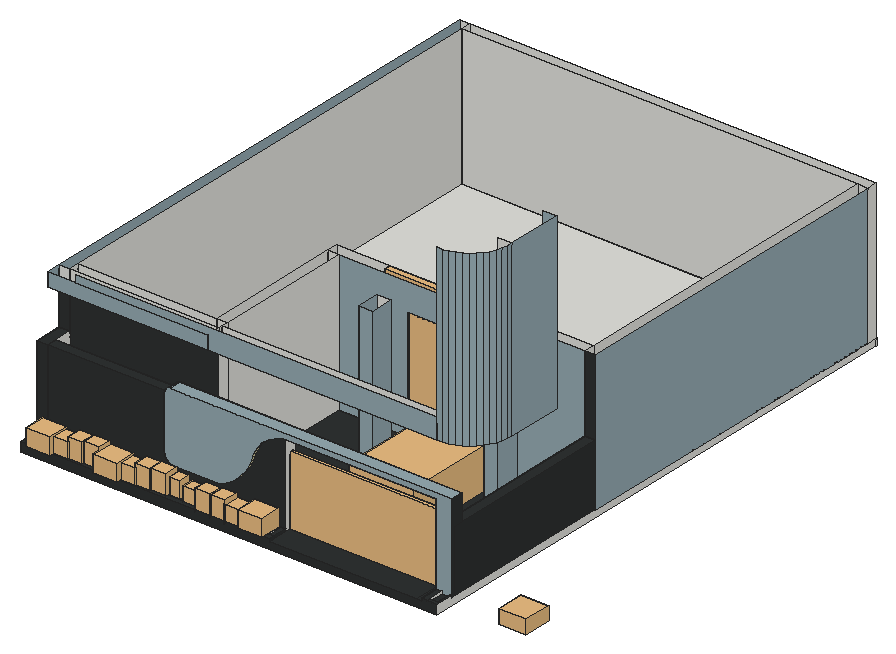
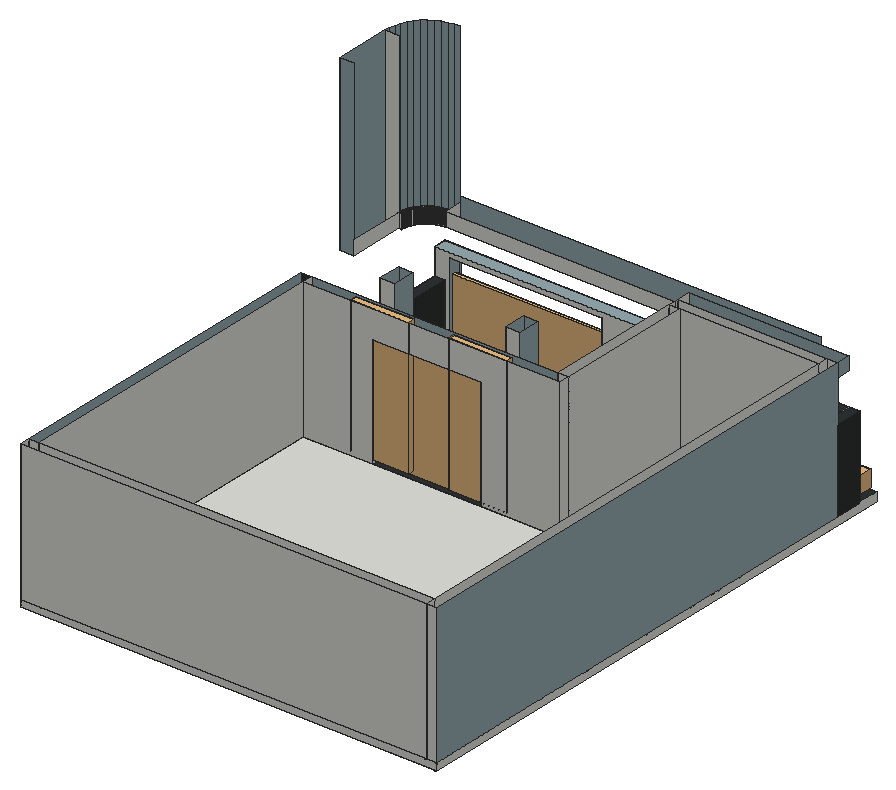
# SketchUp Ruby script. Lengths in inches.
U = 1.inch
M = Sketchup.active_model
def pt(a) = Geom::Point3d.new(a.map { |v| v * U })
def face(e, loops, mat)
  f = e.add_face(loops[0].map { |a| pt(a) })
  loops[1..].each { |l| e.add_face(l.map { |a| pt(a) }).erase! }
  f.material = f.back_material = mat if mat
  f
end
# faces: each face lists its corners as indices into pts; further lists are holes
def faces(e, pts, list, mat = nil) = list.each { |f| face(e, (f[0].is_a?(Array) ? f : [f]).map { |l| l.map { |i| pts[i] } }, mat) }
# xy, xz, yz: faces in a plane at the given z, y or x. An outline is a flat list of corners, or four numbers for a rectangle; further outlines are holes
def ring(l) = l.size == 4 ? [[l[0], l[1]], [l[2], l[1]], [l[2], l[3]], [l[0], l[3]]] : l.each_slice(2).to_a
def flat(e, list, mat, &to3) = list.each { |f| face(e, (f[0].is_a?(Array) ? f : [f]).map { |l| ring(l).map { |u, v| to3.(u, v) } }, mat) }
def xy(e, z, list, mat = nil) = flat(e, list, mat) { |x, y| [x, y, z] }
def xz(e, y, list, mat = nil) = flat(e, list, mat) { |x, z| [x, y, z] }
def yz(e, x, list, mat = nil) = flat(e, list, mat) { |y, z| [x, y, z] }
def lines(e, pts, list) = list.each { |a, b| e.add_line(pt(pts[a]), pt(pts[b])) }
# prism: a flat outline (further loops are holes) pulled along v
def prism(e, loops, v, mat = nil)
  f = face(e, loops, mat); d = Geom::Vector3d.new(v.map { |x| x * U })
  f.pushpull(f.normal.samedirection?(d) ? d.length : -d.length)
end
def box(e, o, s, mat = nil) = prism(e, [[o, [o[0] + s[0], o[1], o[2]], [o[0] + s[0], o[1] + s[1], o[2]], [o[0], o[1] + s[1], o[2]]]], [0, 0, s[2]], mat)
def at(x, y, z, deg = 0) = Geom::Transformation.translation(pt([x, y, z])) * Geom::Transformation.rotation(ORIGIN, Z_AXIS, deg.degrees)
def axes(o, x, y, z) = Geom::Transformation.new([*x, 0, *y, 0, *z, 0, *pt(o).to_a, 1])
def part(name) = M.definitions.add(name)
# library, detail: a bought-in or finely detailed component or shape, given as its bounding box
def library(name, o, s) = part(name).tap { |d| box(d.entities, o, s) }
def detail(e, o, s) = box(e.add_group.entities, o, s)
def put(e, d, t, mat = nil) = e.add_instance(d, t).tap { |i| i.material = mat if mat }
def group(e, t, mat = nil) = e.add_group.tap { |g| g.transformation = t; g.material = mat if mat }.entities
root = M.entities
M.materials.add("Emissive").color = [234, 228, 175]
M.materials.add("Generic").color = [150, 171, 178]
M.materials.add("Generic\#1").color = [47, 50, 50]
c1 = library("Potted Plant 50-12",[-6.11,-5.26,0],[11.24,10.56,13.41])
c2 = library("Untitled",[332.1875,126.3,0],[192,3,60])
c3 = library("2016+Honda+Civic+LX+Sedan",[0.01,0.03,0.02],[16.17,34.46,10.62])
c4 = library("Window 46-47",[-61.02,-2.17,0],[122.04,4.34,74.02])
c5 = library("Potted Plant 50-23",[-3.4,-3.5,0],[6.8,7,9.93])
c6 = library("Plant 160 012",[-4.91,-4.04,0],[10.03,8.97,14.29])
c7 = library("Erigeron glaucus 001",[-10.99,-11.02,0],[21.02,20.18,22.01])
c8 = library("Erigeron glaucus 004",[-15.59,-14.45,0.01],[31.39,28.46,21.32])
c9 = library("Ficus elastica Belize 002",[-7.92,-8.8125,0.01],[22.14,24.73,36.43])
c10 = library("Curtains 003",[-24.98,-2.79,0.01],[49.96,5.58,117.31])
c11 = library("Dome Light",[-12,-12,0],[24,24,12])
xy(root,-6,[[1.218,0,361.218,474.0625],[1.218,474.0625,361.218,474.3125]])
xy(root,0,[[1.218,18.0625,10.218,42.0625],[10.218,18.0625,216.371,27.0625],[352.218,18.0625,361.218,171.0625],[10.218,27.0625,139.218,42.0625],[1.218,42.0625,10.218,474.0625],
  [10.218,42.0625,139.218,51.0625],[10.218,51.0625,130.218,51.0625,130.218,180.0625,352.218,180.0625,352.218,465.0625,10.218,465.0625],[130.218,51.0625,139.218,171.0625],[130.218,51.0625,139.218,51.0625,139.218,171.0625,199.218,171.0625,199.218,180.0625,130.218,180.0625],[130.218,171.0625,199.218,180.0625],
  [292.218,171.0625,352.218,180.0625],[352.218,171.0625,361.218,465.0625],[10.218,465.0625,361.218,474.0625],[1.218,474.0625,10.218,474.3125],[10.218,474.0625,361.218,474.3125]])
xy(root,0,[[[216.371,0,343.218,0,343.218,27.0625,352.218,27.0625,352.218,171.0625,292.218,171.0625,292.218,180.0625,199.218,180.0625,199.218,171.0625,139.218,171.0625,139.218,27.0625,216.371,27.0625],[194.174,124.131,206.361,143.851],[302.424,124.131,314.611,143.851]],[343.218,0,347.629,27.0625],[352.218,3.359,359.091,16],[10.218,5.216,211.73,18.0625]],"Generic\#1")
xy(root,1.8125,[[1.218,0,10.218,18.0625],[10.218,0,216.371,5.216],[211.73,5.216,216.371,18.0625]],"Generic\#1")
xy(root,2.1875,[[347.629,0,352.218,16],[352.218,0,361.218,3.359],[359.091,3.359,361.218,16]],"Generic\#1")
xy(root,18.134,[[121.177,16,159.058,18.0625]],"Emissive")
xy(root,54.125,[[352.218,18.0625,361.218,27.0625]])
xy(root,54.125,[[352.218,27.0625,361.218,171.0625]],"Generic\#1")
xy(root,72,[[1.218,18.0625,10.218,42.0625],[10.218,18.0625,112.749,27.0625]],"Generic\#1")
xy(root,72.458,[[216.371,16,347.629,18.0625],[216.371,18.0625,347.629,27.0625]],"Generic")
xy(root,76.875,[[118.243,16,361.218,27.0625]],"Generic")
xy(root,96,[[199.218,171.0625,292.218,180.0625]])
xy(root,108,[[139.218,29.933,1.206,30.0625,1.218,42.0625,139.218,41.933],[139.218,29.933,139.218,41.933,139.295,41.933,139.284,29.933],[337.222,41.748,337.218,42.0625,337.222,42.0625]])
xy(root,108,[[139.284,29.933,139.295,41.933,139.218,41.933,139.218,44.654,337.184,44.654,337.184,29.933],[337.218,29.933,337.218,42.0625,337.222,41.748,337.854,41.757,338.49,41.782,339.125,41.823,339.759,41.882,340.391,41.956,341.021,42.048,341.648,42.155,342.273,42.28,342.894,42.42,343.511,42.577,344.123,42.75,344.731,42.938,345.334,43.143,345.931,43.363,346.522,43.599,347.107,43.85,347.685,44.117,348.256,44.398,348.819,44.695,349.375,45.006,349.922,45.331,350.46,45.671,350.989,46.025,351.509,46.392,352.019,46.773,352.519,47.167,353.008,47.574,353.487,47.994,353.954,48.426,354.41,48.87,354.854,49.326,355.287,49.793,355.706,50.272,356.113,50.761,356.507,51.261,356.888,51.771,357.256,52.291,357.609,52.82,357.949,53.358,358.274,53.905,358.585,54.461,358.882,55.024,359.163,55.595,359.43,56.173,359.681,56.758,359.917,57.349,360.137,57.946,360.342,58.549,360.531,59.157,360.703,59.77,360.86,60.386,361,61.007,361.125,61.632,361.232,62.259,361.324,62.889,361.399,63.521,361.457,64.155,361.498,64.79,361.523,65.426,361.532,66.058,361.218,66.0625,373.218,66.0625,373.083,61.296,372.298,56.592,370.876,52.04,368.843,47.726,366.24,43.731,363.114,40.13,359.524,36.991,355.538,34.373,351.231,32.326,346.685,30.887,341.984,30.085],[337.222,41.748,337.222,42.0625,337.218,42.0625,337.184,44.654,337.778,44.662,338.338,44.684,338.897,44.72,339.455,44.772,340.012,44.838,340.567,44.918,341.119,45.013,341.669,45.122,342.215,45.246,342.758,45.384,343.298,45.536,343.833,45.702,344.364,45.882,344.89,46.076,345.41,46.284,345.925,46.505,346.434,46.74,346.937,46.988,347.433,47.249,347.922,47.523,348.403,47.809,348.877,48.108,349.343,48.42,349.801,48.743,350.25,49.078,350.69,49.425,351.121,49.784,351.542,50.153,351.954,50.534,352.355,50.925,352.746,51.326,353.127,51.738,353.496,52.159,353.855,52.59,354.202,53.03,354.537,53.479,354.861,53.937,355.172,54.403,355.471,54.877,355.757,55.358,356.031,55.847,356.292,56.343,356.54,56.846,356.775,57.355,356.996,57.87,357.204,58.391,357.398,58.916,357.578,59.447,357.744,59.982,357.896,60.522,358.034,61.065,358.158,61.612,358.267,62.161,358.362,62.714,358.442,63.268,358.508,63.825,358.56,64.383,358.596,64.942,358.618,65.502,358.626,66.096,361.218,66.0625,361.532,66.058,361.523,65.426,361.498,64.79,361.457,64.155,361.399,63.521,361.324,62.889,361.232,62.259,361.125,61.632,361,61.007,360.86,60.386,360.703,59.77,360.531,59.157,360.342,58.549,360.137,57.946,359.917,57.349,359.681,56.758,359.43,56.173,359.163,55.595,358.882,55.024,358.585,54.461,358.274,53.905,357.949,53.358,357.609,52.82,357.256,52.291,356.888,51.771,356.507,51.261,356.113,50.761,355.706,50.272,355.287,49.793,354.854,49.326,354.41,48.87,353.954,48.426,353.487,47.994,353.008,47.574,352.519,47.167,352.019,46.773,351.509,46.392,350.989,46.025,350.46,45.671,349.922,45.331,349.375,45.006,348.819,44.695,348.256,44.398,347.685,44.117,347.107,43.85,346.522,43.599,345.931,43.363,345.334,43.143,344.731,42.938,344.123,42.75,343.511,42.577,342.894,42.42,342.273,42.28,341.648,42.155,341.021,42.048,340.391,41.956,339.759,41.882,339.125,41.823,338.49,41.782,337.854,41.757],[361.218,66.0625,373.218,114.0625]],"Generic")
xz(root,0,[[1.218,-6,361.218,-6,361.218,2.1875,347.629,2.1875,347.629,0,216.371,0,216.371,1.8125,1.218,1.8125]],"Generic\#1")
xz(root,3.359,[[352.218,0,359.091,2.1875]])
xz(root,5.216,[[10.218,0,211.73,1.8125]])
xz(root,16,[[352.218,0,359.091,0,359.091,2.1875,361.218,2.1875,361.218,76.875,118.243,76.875,117.575,76.835,116.917,76.714,116.279,76.515,115.669,76.24,115.096,75.893,114.57,75.481,114.098,75.007,113.686,74.48,113.34,73.907,113.067,73.297,112.868,72.658,112.749,72,112.749,26.562,112.821,25.462,113.036,24.381,113.391,23.337,113.878,22.348,114.491,21.431,115.218,20.602,116.046,19.875,116.963,19.263,117.952,18.775,118.996,18.421,120.077,18.206,121.177,18.134,159.058,18.134,162.568,19.401,165.964,20.947,169.225,22.762,172.328,24.833,175.255,27.148,177.986,29.69,180.503,32.445,182.791,35.393,184.833,38.516,186.617,41.793,188.131,45.204,189.366,48.725,190.427,51.694,191.756,54.554,193.342,57.278,195.173,59.846,197.232,62.234,199.502,64.422,201.964,66.392,204.596,68.127,207.378,69.613,210.284,70.837,213.29,71.788,216.371,72.458,347.629,72.458,347.629,2.1875,352.218,2.1875]],"Generic")
xz(root,18.0625,[[1.218,0,10.218,1.8125],[211.73,0,216.371,1.8125],[352.218,0,361.218,54.125]])
xz(root,18.0625,[[10.218,0,211.73,0,211.73,1.8125,216.371,1.8125,216.371,72.458,213.29,71.788,210.284,70.837,207.378,69.613,204.596,68.127,201.964,66.392,199.502,64.422,197.232,62.234,195.173,59.846,193.342,57.278,191.756,54.554,190.427,51.694,189.366,48.725,188.131,45.204,186.617,41.793,184.833,38.516,182.791,35.393,180.503,32.445,177.986,29.69,175.255,27.148,172.328,24.833,169.225,22.762,165.964,20.947,162.568,19.401,159.058,18.134,121.177,18.134,120.077,18.206,118.996,18.421,117.952,18.775,116.963,19.263,116.046,19.875,115.218,20.602,114.491,21.431,113.878,22.348,113.391,23.337,113.036,24.381,112.821,25.462,112.749,26.562,112.749,72,10.218,72],[1.218,1.8125,10.218,72]],"Generic\#1")
xz(root,27.0625,[[10.218,0,10.218,72,112.749,72,112.868,72.658,113.067,73.297,113.34,73.907,113.686,74.48,114.098,75.007,114.57,75.481,115.096,75.893,115.669,76.24,116.279,76.515,116.917,76.714,117.575,76.835,118.243,76.875,361.218,76.875,361.218,54.125,352.218,54.125,352.218,0,347.629,0,347.629,72.458,216.371,72.458,216.371,0]])
xz(root,29.933,[[139.218,108,139.284,120]])
xz(root,29.933,[[139.284,108,337.184,108,337.184,120,337.218,120,337.218,126,25.218,126,25.218,120,139.284,120]],"Generic")
xz(root,42.0625,[[1.218,0,10.218,72],[1.218,108,10.218,120],[10.218,108,139.218,120]])
xz(root,42.0625,[[10.218,0,139.218,108],[1.218,72,10.218,108]],"Generic\#1")
xz(root,44.654,[[139.218,108,337.184,120]])
xz(root,51.0625,[[10.218,0,130.218,120],[130.218,0,139.218,120]])
xz(root,66.0625,[[361.218,108,373.218,257]])
xz(root,114.0625,[[361.218,108,373.218,257]],"Generic")
xz(root,124.131,[[194.174,0,206.361,120],[302.424,0,314.611,120]],"Generic")
xz(root,143.851,[[194.174,0,206.361,120],[302.424,0,314.611,120]])
xz(root,171.0625,[[130.218,0,139.218,120],[352.218,0,361.218,54.125]])
xz(root,171.0625,[[139.218,0,199.218,0,199.218,96,292.218,96,292.218,0,352.218,0,352.218,120,139.218,120]],"Generic")
xz(root,171.0625,[[352.218,54.125,361.218,120]],"Generic\#1")
xz(root,180.0625,[[130.218,0,130.218,120,352.218,120,352.218,0,292.218,0,292.218,96,199.218,96,199.218,0]])
xz(root,465.0625,[[10.218,0,352.218,120],[352.218,0,361.218,120]])
xz(root,474.0625,[[1.218,0,10.218,120],[10.218,0,361.218,120]])
xz(root,474.3125,[[1.218,-6,361.218,0]])
yz(root,1.218,[[0,-6,0,1.8125,18.0625,1.8125,18.0625,0,474.0625,0,474.0625,-6],[474.0625,-6,474.3125,0]])
yz(root,1.218,[[42.0625,0,474.0625,120]],"Generic")
yz(root,1.218,[[18.0625,0,42.0625,72]],"Generic\#1")
yz(root,10.218,[[5.216,0,18.0625,1.8125],[18.0625,0,27.0625,72],[27.0625,0,42.0625,72],[42.0625,0,51.0625,120],[51.0625,0,465.0625,120],
  [465.0625,0,474.0625,120]])
yz(root,112.749,[[16,26.562,18.0625,72]],"Emissive")
yz(root,130.218,[[51.0625,0,171.0625,120],[171.0625,0,180.0625,120]])
yz(root,139.218,[[42.0625,0,51.0625,0,51.0625,120,44.654,120,44.654,108,42.0625,108],[51.0625,0,171.0625,120],[29.933,108,42.0625,120],[42.0625,108,44.654,120]])
yz(root,194.174,[[124.131,0,143.851,120]],"Generic")
yz(root,199.218,[[171.0625,0,180.0625,96]])
yz(root,206.361,[[124.131,0,143.851,120]],"Generic")
yz(root,211.73,[[5.216,0,18.0625,1.8125]])
yz(root,216.371,[[18.0625,0,27.0625,72.458]])
yz(root,216.371,[[0,0,5.216,1.8125],[5.216,0,18.0625,1.8125]],"Generic\#1")
yz(root,292.218,[[171.0625,0,180.0625,96]])
yz(root,302.424,[[124.131,0,143.851,120]],"Generic")
yz(root,314.611,[[124.131,0,143.851,120]],"Generic")
yz(root,337.184,[[29.933,108,44.654,120]])
yz(root,337.218,[[29.933,108,42.0625,120]])
yz(root,337.222,[[41.748,108,42.0625,120]])
yz(root,347.629,[[16,0,18.0625,72.458],[18.0625,0,27.0625,72.458]],"Generic")
yz(root,347.629,[[0,0,16,2.1875]],"Generic\#1")
yz(root,352.218,[[3.359,0,16,2.1875],[18.0625,0,27.0625,54.125],[171.0625,0,180.0625,120],[180.0625,0,465.0625,120]])
yz(root,352.218,[[27.0625,0,171.0625,54.125]],"Generic\#1")
yz(root,359.091,[[3.359,0,16,2.1875]],"Generic\#1")
yz(root,361.218,[[0,-6,474.0625,-6,474.0625,0,16,0,16,2.1875,0,2.1875],[474.0625,-6,474.3125,0],[465.0625,0,474.0625,120],[66.0625,108,114.0625,120]])
yz(root,361.218,[[171.0625,0,465.0625,120]],"Generic")
yz(root,361.218,[[16,0,18.0625,0,18.0625,54.125,27.0625,54.125,27.0625,76.875,16,76.875],[18.0625,0,171.0625,54.125]],"Generic\#1")
yz(root,373.218,[[66.0625,108,114.0625,257]],"Generic")
p = [[120.077,18.0625,18.206],[121.177,18.0625,18.134],[121.177,16,18.134],[120.077,16,18.206],[159.058,18.0625,18.134],[162.568,18.0625,19.401],
  [162.568,16,19.401],[159.058,16,18.134],[118.996,18.0625,18.421],[118.996,16,18.421],[117.952,18.0625,18.775],[117.952,16,18.775],
  [116.963,18.0625,19.263],[116.963,16,19.263],[116.046,18.0625,19.875],[116.046,16,19.875],[165.964,18.0625,20.947],[165.964,16,20.947],
  [115.218,18.0625,20.602],[115.218,16,20.602],[114.491,18.0625,21.431],[114.491,16,21.431],[169.225,18.0625,22.762],[169.225,16,22.762],
  [113.878,18.0625,22.348],[113.878,16,22.348],[113.391,18.0625,23.337],[113.391,16,23.337],[172.328,18.0625,24.833],[172.328,16,24.833],
  [113.036,18.0625,24.381],[113.036,16,24.381],[112.821,18.0625,25.462],[112.821,16,25.462],[175.255,18.0625,27.148],[175.255,16,27.148],
  [112.749,18.0625,26.562],[112.749,16,26.562],[177.986,18.0625,29.69],[177.986,16,29.69],[180.503,18.0625,32.445],[180.503,16,32.445],
  [182.791,18.0625,35.393],[182.791,16,35.393],[184.833,18.0625,38.516],[184.833,16,38.516],[186.617,18.0625,41.793],[186.617,16,41.793],
  [188.131,18.0625,45.204],[188.131,16,45.204],[189.366,18.0625,48.725],[189.366,16,48.725],[190.427,18.0625,51.694],[190.427,16,51.694],
  [191.756,18.0625,54.554],[191.756,16,54.554],[193.342,18.0625,57.278],[193.342,16,57.278],[195.173,18.0625,59.846],[195.173,16,59.846],
  [197.232,18.0625,62.234],[197.232,16,62.234],[199.502,18.0625,64.422],[199.502,16,64.422],[201.964,18.0625,66.392],[201.964,16,66.392],
  [204.596,18.0625,68.127],[204.596,16,68.127],[207.378,18.0625,69.613],[207.378,16,69.613],[210.284,18.0625,70.837],[210.284,16,70.837],
  [213.29,18.0625,71.788],[213.29,16,71.788],[216.371,18.0625,72.458],[216.371,16,72.458],[112.749,27.0625,72],[112.749,18.0625,72],
  [112.749,16,72],[112.868,16,72.658],[112.868,27.0625,72.658],[113.067,16,73.297],[113.067,27.0625,73.297],[113.34,16,73.907],
  [113.34,27.0625,73.907],[113.686,16,74.48],[113.686,27.0625,74.48],[114.098,16,75.007],[114.098,27.0625,75.007],[114.57,16,75.481],
  [114.57,27.0625,75.481],[115.096,16,75.893],[115.096,27.0625,75.893],[115.669,16,76.24],[115.669,27.0625,76.24],[116.279,16,76.515],
  [116.279,27.0625,76.515],[116.917,16,76.714],[116.917,27.0625,76.714],[117.575,16,76.835],[117.575,27.0625,76.835],[118.243,16,76.875],
  [118.243,27.0625,76.875],[1.206,30.0625,108],[139.218,29.933,108],[139.218,29.933,120],[25.218,30.04,120],[10.218,30.054,120],
  [1.218,30.0625,120],[1.206,30.0625,120],[139.295,41.933,108],[139.295,41.933,120],[139.284,29.933,120],[139.284,29.933,108],
  [337.218,29.933,126],[337.218,29.933,120],[337.218,29.933,108],[341.984,30.085,108],[341.984,30.085,257],[337.218,29.933,257],
  [337.218,29.933,132],[1.218,42.0625,120],[1.218,42.0625,108],[346.685,30.887,108],[346.685,30.887,257],[351.231,32.326,108],
  [351.231,32.326,257],[355.538,34.373,108],[355.538,34.373,257],[359.524,36.991,108],[359.524,36.991,257],[363.114,40.13,108],
  [363.114,40.13,257],[366.24,43.731,108],[366.24,43.731,257],[337.854,41.757,120],[337.222,41.748,120],[337.222,41.748,108],
  [337.854,41.757,108],[337.218,42.0625,120],[337.218,42.0625,108],[338.49,41.782,108],[338.49,41.782,120],[339.125,41.823,108],
  [339.125,41.823,120],[339.759,41.882,108],[339.759,41.882,120],[340.391,41.956,108],[340.391,41.956,120],[341.021,42.048,108],
  [341.021,42.048,120],[341.648,42.155,108],[341.648,42.155,120],[337.184,44.654,108],[337.184,44.654,120],[342.273,42.28,108],
  [342.273,42.28,120],[342.894,42.42,108],[342.894,42.42,120],[343.511,42.577,108],[343.511,42.577,120],[344.123,42.75,108],
  [344.123,42.75,120],[344.731,42.938,108],[344.731,42.938,120],[345.334,43.143,108],[345.334,43.143,120],[345.931,43.363,108],
  [345.931,43.363,120],[346.522,43.599,108],[346.522,43.599,120],[347.107,43.85,108],[347.107,43.85,120],[368.843,47.726,108],
  [368.843,47.726,257],[347.685,44.117,108],[347.685,44.117,120],[348.256,44.398,108],[348.256,44.398,120],[348.819,44.695,108],
  [348.819,44.695,120],[337.778,44.662,108],[337.778,44.662,120],[338.338,44.684,120],[338.338,44.684,108],[338.897,44.72,120],
  [338.897,44.72,108],[339.455,44.772,120],[339.455,44.772,108],[349.375,45.006,108],[349.375,45.006,120],[340.012,44.838,120],
  [340.012,44.838,108],[340.567,44.918,120],[340.567,44.918,108],[341.119,45.013,120],[341.119,45.013,108],[341.669,45.122,120],
  [341.669,45.122,108],[349.922,45.331,108],[349.922,45.331,120],[342.215,45.246,120],[342.215,45.246,108],[342.758,45.384,120],
  [342.758,45.384,108],[350.46,45.671,108],[350.46,45.671,120],[343.298,45.536,120],[343.298,45.536,108],[343.833,45.702,120],
  [343.833,45.702,108],[344.364,45.882,120],[344.364,45.882,108],[350.989,46.025,108],[350.989,46.025,120],[344.89,46.076,120],
  [344.89,46.076,108],[351.509,46.392,108],[351.509,46.392,120],[345.41,46.284,120],[345.41,46.284,108],[345.925,46.505,120],
  [345.925,46.505,108],[352.019,46.773,108],[352.019,46.773,120],[346.434,46.74,120],[346.434,46.74,108],[346.937,46.988,120],
  [346.937,46.988,108],[352.519,47.167,108],[352.519,47.167,120],[347.433,47.249,120],[347.433,47.249,108],[347.922,47.523,120],
  [347.922,47.523,108],[353.008,47.574,108],[353.008,47.574,120],[348.403,47.809,120],[348.403,47.809,108],[353.487,47.994,108],
  [353.487,47.994,120],[370.876,52.04,108],[370.876,52.04,257],[348.877,48.108,120],[348.877,48.108,108],[353.954,48.426,108],
  [353.954,48.426,120],[349.343,48.42,120],[349.343,48.42,108],[349.801,48.743,120],[349.801,48.743,108],[354.41,48.87,108],
  [354.41,48.87,120],[350.25,49.078,120],[350.25,49.078,108],[354.854,49.326,108],[354.854,49.326,120],[350.69,49.425,120],
  [350.69,49.425,108],[355.287,49.793,108],[355.287,49.793,120],[351.121,49.784,120],[351.121,49.784,108],[351.542,50.153,120],
  [351.542,50.153,108],[355.706,50.272,108],[355.706,50.272,120],[351.954,50.534,120],[351.954,50.534,108],[356.113,50.761,108],
  [356.113,50.761,120],[352.355,50.925,120],[352.355,50.925,108],[356.507,51.261,108],[356.507,51.261,120],[352.746,51.326,120],
  [352.746,51.326,108],[353.127,51.738,120],[353.127,51.738,108],[356.888,51.771,108],[356.888,51.771,120],[353.496,52.159,120],
  [353.496,52.159,108],[357.256,52.291,108],[357.256,52.291,120],[372.298,56.592,108],[372.298,56.592,257],[353.855,52.59,120],
  [353.855,52.59,108],[357.609,52.82,108],[357.609,52.82,120],[354.202,53.03,120],[354.202,53.03,108],[357.949,53.358,108],
  [357.949,53.358,120],[354.537,53.479,120],[354.537,53.479,108],[358.274,53.905,108],[358.274,53.905,120],[354.861,53.937,120],
  [354.861,53.937,108],[355.172,54.403,120],[355.172,54.403,108],[358.585,54.461,108],[358.585,54.461,120],[355.471,54.877,120],
  [355.471,54.877,108],[358.882,55.024,108],[358.882,55.024,120],[355.757,55.358,120],[355.757,55.358,108],[359.163,55.595,108],
  [359.163,55.595,120],[356.031,55.847,120],[356.031,55.847,108],[359.43,56.173,108],[359.43,56.173,120],[356.292,56.343,120],
  [356.292,56.343,108],[359.681,56.758,108],[359.681,56.758,120],[356.54,56.846,120],[356.54,56.846,108],[373.083,61.296,108],
  [373.083,61.296,257],[356.775,57.355,120],[356.775,57.355,108],[359.917,57.349,108],[359.917,57.349,120],[360.137,57.946,108],
  [360.137,57.946,120],[356.996,57.87,120],[356.996,57.87,108],[357.204,58.391,120],[357.204,58.391,108],[360.342,58.549,108],
  [360.342,58.549,120],[357.398,58.916,120],[357.398,58.916,108],[360.531,59.157,108],[360.531,59.157,120],[357.578,59.447,120],
  [357.578,59.447,108],[360.703,59.77,108],[360.703,59.77,120],[357.744,59.982,120],[357.744,59.982,108],[360.86,60.386,108],
  [360.86,60.386,120],[357.896,60.522,120],[357.896,60.522,108],[361,61.007,108],[361,61.007,120],[358.034,61.065,120],
  [358.034,61.065,108],[361.125,61.632,108],[361.125,61.632,120],[358.158,61.612,120],[358.158,61.612,108],[373.218,66.0625,108],
  [373.218,66.0625,257],[358.267,62.161,120],[358.267,62.161,108],[361.232,62.259,108],[361.232,62.259,120],[358.362,62.714,120],
  [358.362,62.714,108],[361.324,62.889,108],[361.324,62.889,120],[358.442,63.268,120],[358.442,63.268,108],[361.399,63.521,108],
  [361.399,63.521,120],[358.508,63.825,120],[358.508,63.825,108],[361.457,64.155,108],[361.457,64.155,120],[358.56,64.383,120],
  [358.56,64.383,108],[361.498,64.79,108],[361.498,64.79,120],[358.596,64.942,120],[358.596,64.942,108],[361.523,65.426,108],
  [361.523,65.426,120],[358.618,65.502,120],[358.618,65.502,108],[361.532,66.058,108],[361.532,66.058,120],[358.626,66.096,120],
  [358.626,66.096,108],[361.218,66.0625,120],[361.218,66.0625,108]]
faces(root,p,[[0,1,2,3],[4,5,6,7],[8,0,3,9],[10,8,9,11],[12,10,11,13],[14,12,13,15],[5,16,17,6],[18,14,15,19],
  [20,18,19,21],[16,22,23,17],[24,20,21,25],[26,24,25,27],[22,28,29,23],[30,26,27,31],[32,30,31,33],[28,34,35,29],
  [36,32,33,37],[34,38,39,35],[38,40,41,39],[40,42,43,41],[42,44,45,43],[44,46,47,45],[46,48,49,47],[48,50,51,49],
  [50,52,53,51],[52,54,55,53],[54,56,57,55],[56,58,59,57],[58,60,61,59],[60,62,63,61],[62,64,65,63],[64,66,67,65],
  [66,68,69,67],[68,70,71,69],[70,72,73,71],[72,74,75,73]],"Emissive")
faces(root,p,[[76,77,78,79,80],[80,79,81,82],[82,81,83,84],[84,83,85,86],[86,85,87,88],[88,87,89,90],[90,89,91,92],[92,91,93,94],
  [94,93,95,96],[96,95,97,98],[98,97,99,100],[100,99,101,102],[103,104,105,106,107,108,109],[114,115,116,117,118,119,120],[121,122,103,109],[118,117,123,124],
  [124,123,125,126],[126,125,127,128],[128,127,129,130],[130,129,131,132],[132,131,133,134],[134,133,173,174],[174,173,241,242],[242,241,285,286],
  [286,285,323,324],[324,323,359,360]],"Generic")
faces(root,p,[[110,111,112,113],[135,136,137,138],[136,139,140,137],[135,138,141,142],[142,141,143,144],[144,143,145,146],[146,145,147,148],[148,147,149,150],
  [150,149,151,152],[153,140,139,154],[152,151,155,156],[156,155,157,158],[158,157,159,160],[160,159,161,162],[162,161,163,164],[164,163,165,166],
  [166,165,167,168],[168,167,169,170],[170,169,171,172],[172,171,175,176],[176,175,177,178],[178,177,179,180],[181,153,154,182],[181,182,183,184],
  [184,183,185,186],[186,185,187,188],[180,179,189,190],[188,187,191,192],[192,191,193,194],[194,193,195,196],[196,195,197,198],[190,189,199,200],
  [198,197,201,202],[202,201,203,204],[200,199,205,206],[204,203,207,208],[208,207,209,210],[210,209,211,212],[206,205,213,214],[212,211,215,216],
  [214,213,217,218],[216,215,219,220],[220,219,221,222],[218,217,223,224],[222,221,225,226],[226,225,227,228],[224,223,229,230],[228,227,231,232],
  [232,231,233,234],[230,229,235,236],[234,233,237,238],[236,235,239,240],[238,237,243,244],[240,239,245,246],[244,243,247,248],[248,247,249,250],
  [246,245,251,252],[250,249,253,254],[252,251,255,256],[254,253,257,258],[256,255,259,260],[258,257,261,262],[262,261,263,264],[260,259,265,266],
  [264,263,267,268],[266,265,269,270],[268,267,271,272],[270,269,273,274],[272,271,275,276],[276,275,277,278],[274,273,279,280],[278,277,281,282],
  [280,279,283,284],[282,281,287,288],[284,283,289,290],[288,287,291,292],[290,289,293,294],[292,291,295,296],[294,293,297,298],[296,295,299,300],
  [300,299,301,302],[298,297,303,304],[302,301,305,306],[304,303,307,308],[306,305,309,310],[308,307,311,312],[310,309,313,314],[312,311,315,316],
  [314,313,317,318],[316,315,319,320],[318,317,321,322],[322,321,325,326],[320,319,327,328],[328,327,329,330],[326,325,331,332],[332,331,333,334],
  [330,329,335,336],[334,333,337,338],[336,335,339,340],[338,337,341,342],[340,339,343,344],[342,341,345,346],[344,343,347,348],[346,345,349,350],
  [348,347,351,352],[350,349,353,354],[352,351,355,356],[354,353,357,358],[358,357,361,362],[356,355,363,364],[362,361,365,366],[364,363,367,368],
  [366,365,369,370],[368,367,371,372],[370,369,373,374],[372,371,375,376],[374,373,377,378],[376,375,379,380],[378,377,381,382],[380,379,383,384],
  [382,381,385,386],[384,383,387,388],[386,385,389,390],[389,391,392,390],[391,388,387,392]])
put(root,c1,at(144.42,9.72,0))
put(root,c2,axes([-10.72,-103.73,0],[0.68364,0,0],[0,1,0],[0,0,1]))
put(root,c3,axes([286.3125,163.9,-0.07],[-3.45512,0,0],[0,-2.7641,0],[0,0,3.34456]))
put(root,c4,axes([245.99,173.21,0],[0.75761,0,0],[0,1,0],[0,0,1.30094]))
put(root,c5,axes([171.56,6.83,0],[-1.83,0,0],[0,-1.83,0],[0,0,1.83]))
put(root,c5,axes([46.39,8.82,0],[1.83,0,0],[0,1.83,0],[0,0,1.83]))
put(root,c5,axes([104.52,8.82,0],[1.83,0,0],[0,1.83,0],[0,0,1.83]))
put(root,c6,axes([158.6,6.69,0],[-1.3,0,0],[0,-1.3,0],[0,0,1.3]))
put(root,c6,axes([59.35,8.96,0],[1.3,0,0],[0,1.3,0],[0,0,1.3]))
put(root,c6,axes([117.47,8.96,0],[1.3,0,0],[0,1.3,0],[0,0,1.3]))
put(root,c7,axes([183.71,6.62,0],[-0.67,0,0],[0,-0.67,0],[0,0,0.67]))
put(root,c7,axes([34.24,9.03,0],[0.67,0,0],[0,0.67,0],[0,0,0.67]))
put(root,c7,axes([92.36,9.03,0],[0.67,0,0],[0,0.67,0],[0,0,0.67]))
put(root,c8,axes([200.05,8.45,1.63],[-0.66,0,0],[0,-0.66,0],[0,0,0.66]))
put(root,c8,axes([17.9,7.2,1.63],[0.66,0,0],[0,0.66,0],[0,0,0.66]))
put(root,c8,axes([76.02,7.2,1.63],[0.66,0,0],[0,0.66,0],[0,0,0.66]))
put(root,c9,axes([129.08,8.62,1.82],[0.4,0,0],[0,0.4,0],[0,0,0.4]))
put(root,c10,at(286.13,177.25,3.05))
put(root,c10,at(201.38,177.25,3.05))
put(root,c11,at(460.52,-30.96,36.61))
